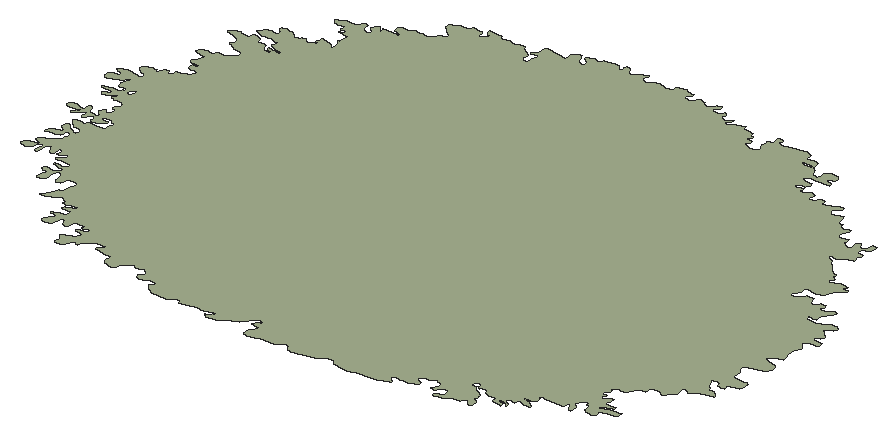
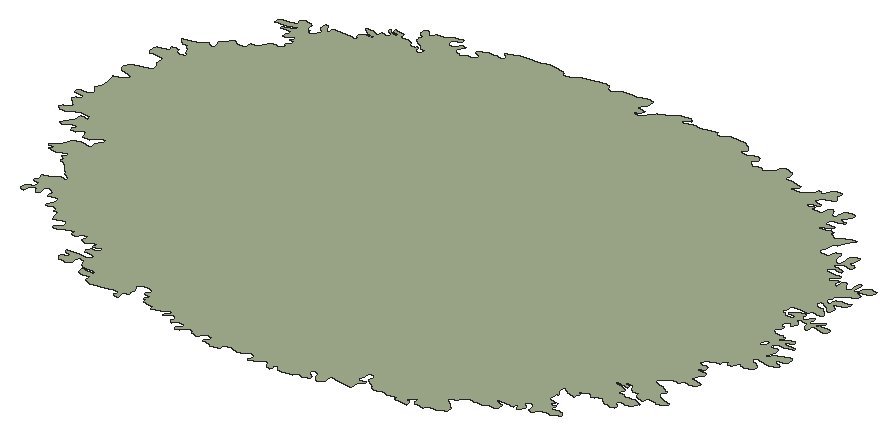
# SketchUp Ruby script. Lengths in inches.
U = 1.inch
M = Sketchup.active_model
def pt(a) = Geom::Point3d.new(a.map { |v| v * U })
def face(e, loops, mat)
  f = e.add_face(loops[0].map { |a| pt(a) })
  loops[1..].each { |l| e.add_face(l.map { |a| pt(a) }).erase! }
  f.material = f.back_material = mat if mat
  f
end
# faces: each face lists its corners as indices into pts; further lists are holes
def faces(e, pts, list, mat = nil) = list.each { |f| face(e, (f[0].is_a?(Array) ? f : [f]).map { |l| l.map { |i| pts[i] } }, mat) }
# xy, xz, yz: faces in a plane at the given z, y or x. An outline is a flat list of corners, or four numbers for a rectangle; further outlines are holes
def ring(l) = l.size == 4 ? [[l[0], l[1]], [l[2], l[1]], [l[2], l[3]], [l[0], l[3]]] : l.each_slice(2).to_a
def flat(e, list, mat, &to3) = list.each { |f| face(e, (f[0].is_a?(Array) ? f : [f]).map { |l| ring(l).map { |u, v| to3.(u, v) } }, mat) }
def xy(e, z, list, mat = nil) = flat(e, list, mat) { |x, y| [x, y, z] }
def xz(e, y, list, mat = nil) = flat(e, list, mat) { |x, z| [x, y, z] }
def yz(e, x, list, mat = nil) = flat(e, list, mat) { |y, z| [x, y, z] }
def lines(e, pts, list) = list.each { |a, b| e.add_line(pt(pts[a]), pt(pts[b])) }
# prism: a flat outline (further loops are holes) pulled along v
def prism(e, loops, v, mat = nil)
  f = face(e, loops, mat); d = Geom::Vector3d.new(v.map { |x| x * U })
  f.pushpull(f.normal.samedirection?(d) ? d.length : -d.length)
end
def box(e, o, s, mat = nil) = prism(e, [[o, [o[0] + s[0], o[1], o[2]], [o[0] + s[0], o[1] + s[1], o[2]], [o[0], o[1] + s[1], o[2]]]], [0, 0, s[2]], mat)
def at(x, y, z, deg = 0) = Geom::Transformation.translation(pt([x, y, z])) * Geom::Transformation.rotation(ORIGIN, Z_AXIS, deg.degrees)
def axes(o, x, y, z) = Geom::Transformation.new([*x, 0, *y, 0, *z, 0, *pt(o).to_a, 1])
def part(name) = M.definitions.add(name)
# library, detail: a bought-in or finely detailed component or shape, given as its bounding box
def library(name, o, s) = part(name).tap { |d| box(d.entities, o, s) }
def detail(e, o, s) = box(e.add_group.entities, o, s)
def put(e, d, t, mat = nil) = e.add_instance(d, t).tap { |i| i.material = mat if mat }
def group(e, t, mat = nil) = e.add_group.tap { |g| g.transformation = t; g.material = mat if mat }.entities
root = M.entities
M.materials.add("Boxwoodplan").color = [166, 177, 144]
xy(root,9.058,[[[69.667,67.129,69.556,67.133,69.461,67.159,69.405,67.215,69.403,67.317,69.429,67.382,69.493,67.445,69.542,67.509,69.6,67.606,69.414,67.635,69.324,67.644,69.344,67.732,69.43,67.79,69.461,67.8,69.456,67.846,69.367,67.877,69.251,67.837,69.154,67.706,69.011,67.551,68.85,67.464,68.745,67.441,68.684,67.416,68.668,67.373,68.524,67.281,68.33,67.251,68.241,67.26,68.161,67.306,68.161,67.328,68.206,67.359,68.297,67.437,68.365,67.483,68.276,67.498,68.163,67.48,68.043,67.436,67.947,67.445,67.85,67.454,67.753,67.447,67.626,67.403,67.426,67.356,67.337,67.349,67.299,67.443,67.291,67.465,67.224,67.473,67.135,67.454,66.966,67.336,66.766,67.328,66.536,67.353,66.369,67.446,66.228,67.61,66.411,67.702,66.311,67.756,66.175,67.772,66.049,67.749,65.977,67.697,65.896,67.672,65.78,67.738,65.738,67.806,65.826,67.847,65.852,67.907,65.857,67.957,65.816,68.009,65.744,68.085,65.658,68.117,65.571,68.064,65.505,68.038,65.449,68.08,65.432,68.103,65.408,68.121,65.379,68.111,65.299,68.058,65.228,68.01,65.152,67.923,65.14,67.79,65.069,67.749,65.019,67.723,64.959,67.725,64.86,67.746,64.773,67.793,64.729,67.861,64.721,67.951,64.73,68.018,64.743,68.04,64.724,68.08,64.51,68.1,64.578,68.135,64.552,68.136,64.459,68.13,64.289,68.146,64.212,68.173,64.195,68.206,64.21,68.224,64.335,68.314,64.333,68.371,64.248,68.393,64.089,68.39,63.958,68.319,63.861,68.233,63.786,68.199,63.739,68.172,63.738,68.154,63.774,68.101,63.758,68.046,63.688,68.081,63.624,68.121,63.563,68.072,63.541,68.017,63.509,67.904,63.462,67.855,63.389,67.822,63.298,67.816,63.228,67.841,63.209,67.874,63.216,67.892,63.237,67.932,63.259,67.991,63.228,68.048,63.127,68.149,63.241,68.229,63.302,68.269,63.382,68.285,63.449,68.315,63.504,68.37,63.589,68.476,63.517,68.503,63.4375,68.511,63.305,68.53,63.267,68.565,63.274,68.584,63.349,68.62,63.511,68.657,63.553,68.709,63.548,68.748,63.522,68.764,63.372,68.711,63.326,68.732,63.327,68.752,63.35,68.814,63.189,68.825,63.108,68.833,63.054,68.826,63.047,68.806,63.031,68.71,63.016,68.642,62.974,68.591,62.927,68.578,62.908,68.594,62.849,68.639,62.804,68.757,62.765,68.783,62.738,68.784,62.684,68.777,62.677,68.757,62.675,68.641,62.621,68.523,62.56,68.449,62.48,68.419,62.401,68.422,62.355,68.448,62.322,68.506,62.322,68.564,62.376,68.677,62.49,68.784,62.51,68.803,62.497,68.823,62.47,68.829,62.39,68.847,62.309,68.86,62.282,68.875,62.289,68.895,62.309,68.914,62.458,68.982,62.62,69.005,62.662,69.108,62.635,69.169,62.588,69.191,62.561,69.187,62.398,69.168,62.357,69.2,62.364,69.22,62.391,69.279,62.549,69.334,62.721,69.403,62.769,69.442,62.756,69.463,62.659,69.436,62.488,69.417,62.344,69.372,62.255,69.386,62.228,69.392,62.234,69.412,62.255,69.426,62.31,69.47,62.282,69.507,62.255,69.503,62.172,69.511,62.117,69.56,62.103,69.601,62.076,69.597,61.993,69.575,61.836,69.489,61.687,69.413,61.613,69.38,61.558,69.392,61.571,69.412,61.59,69.452,61.617,69.469,61.641,69.55,61.691,69.65,61.723,69.759,61.774,69.812,61.847,69.852,61.891,69.972,61.913,70.112,61.933,70.227,61.929,70.285,61.884,70.321,61.803,70.335,61.717,70.335,61.643,70.31,61.633,70.245,61.634,70.184,61.601,70.124,61.513,70.087,61.456,70.096,61.418,70.155,61.407,70.216,61.381,70.337,61.376,70.4,61.335,70.453,61.308,70.475,61.27,70.491,61.211,70.479,61.177,70.46,61.175,70.428,61.167,70.366,61.17,70.229,61.195,70.167,61.187,70.103,61.136,70.038,61.088,70.01,61.05,69.998,61.012,70.003,60.97,70.011,60.952,70.039,60.948,70.166,60.969,70.223,61.014,70.276,61.03,70.306,61.022,70.334,60.965,70.34,60.883,70.346,60.846,70.362,60.823,70.39,60.82,70.453,60.835,70.483,60.87,70.499,61.042,70.472,61.121,70.497,61.17,70.526,61.231,70.573,61.244,70.636,61.221,70.662,61.177,70.664,61.1,70.67,61.008,70.681,60.907,70.717,60.888,70.746,60.894,70.76,60.913,70.763,60.973,70.775,61.148,70.761,61.238,70.787,61.25,70.844,61.224,70.907,61.152,70.946,61.073,70.953,60.96,70.946,60.86,70.921,60.777,70.939,60.773,70.968,60.793,70.997,60.84,71.054,60.906,71.11,60.959,71.19,60.951,71.224,60.906,71.241,60.841,71.24,60.723,71.14,60.683,71.141,60.649,71.161,60.671,71.22,60.687,71.287,60.644,71.35,60.604,71.366,60.584,71.367,60.578,71.352,60.582,71.306,60.579,71.164,60.538,71.102,60.499,71.108,60.464,71.131,60.366,71.262,60.342,71.327,60.317,71.355,60.302,71.344,60.246,71.293,60.211,71.234,60.231,71.103,60.236,71.037,60.216,70.971,60.166,70.962,60.132,70.978,60.122,71.023,60.142,71.155,60.151,71.233,60.151,71.27,60.136,71.282,60.121,71.272,60.042,71.237,60.002,71.183,59.993,71.12,59.954,71.077,59.817,70.987,59.777,70.977,59.733,70.986,59.653,71.026,59.633,71.056,59.637,71.089,59.67,71.151,59.767,71.237,59.857,71.263,59.947,71.263,60.042,71.267,59.981,71.318,59.83,71.404,59.813,71.466,59.866,71.503,59.958,71.573,60.077,71.635,60.195,71.709,60.231,71.723,60.257,71.746,60.283,71.789,60.286,71.882,60.319,72.003,60.32,72.065,60.299,72.086,60.277,72.095,60.214,72.109,60.181,72.104,60.177,72.088,60.189,71.996,60.147,71.934,60.099,71.899,60.022,71.871,59.951,71.858,59.79,71.833,59.755,71.839,59.742,71.853,59.742,71.86,59.751,71.901,59.768,71.947,59.81,71.995,59.879,72.042,59.938,72.063,59.996,72.065,60.035,72.068,60.055,72.075,60.078,72.096,60.073,72.121,60.019,72.151,59.951,72.207,59.919,72.264,59.915,72.331,59.928,72.382,59.98,72.426,60.006,72.432,60.017,72.425,60.037,72.411,60.08,72.35,60.129,72.304,60.257,72.226,60.331,72.192,60.366,72.177,60.386,72.184,60.41,72.206,60.417,72.222,60.428,72.263,60.413,72.32,60.37,72.366,60.338,72.389,60.304,72.401,60.244,72.401,60.17,72.404,60.127,72.446,60.041,72.519,59.982,72.569,59.943,72.617,59.944,72.646,59.968,72.671,60.024,72.698,60.059,72.703,60.1,72.7,60.16,72.679,60.222,72.677,60.258,72.684,60.292,72.726,60.341,72.757,60.4,72.764,60.471,72.764,60.625,72.771,60.765,72.792,60.798,72.808,60.799,72.826,60.793,72.868,60.781,72.913,60.792,72.957,60.822,73.06,60.809,73.083,60.786,73.097,60.729,73.126,60.676,73.164,60.603,73.192,60.53,73.195,60.48,73.184,60.459,73.17,60.434,73.119,60.439,73.098,60.45,73.093,60.474,73.088,60.625,73.076,60.651,73.071,60.656,73.0625,60.647,73.046,60.607,73.007,60.562,72.964,60.497,72.928,60.435,72.884,60.363,72.849,60.326,72.852,60.306,72.863,60.281,72.9,60.274,72.995,60.257,73.02,60.275,73.034,60.281,73.077,60.275,73.088,60.264,73.088,60.249,73.087,60.223,73.083,60.191,73.076,60.173,73.065,60.092,72.97,60.06,72.915,60.029,72.892,60.006,72.895,59.98,72.916,59.971,72.932,59.965,72.973,59.994,73.057,59.999,73.102,59.99,73.13,59.97,73.137,59.932,73.128,59.912,73.114,59.866,73.064,59.744,72.957,59.708,72.932,59.682,72.927,59.645,72.935,59.633,72.951,59.724,73.057,59.787,73.102,59.801,73.129,59.8,73.145,59.791,73.152,59.78,73.148,59.765,73.143,59.734,73.131,59.65,73.108,59.483,73.089,59.41,73.096,59.362,73.121,59.34,73.149,59.339,73.165,59.356,73.217,59.404,73.264,59.464,73.281,59.535,73.284,59.609,73.266,59.737,73.223,59.823,73.197,59.834,73.201,59.834,73.22,59.825,73.239,59.8,73.287,59.799,73.342,59.806,73.407,59.818,73.437,59.835,73.45,59.884,73.413,59.923,73.363,59.95,73.317,59.96,73.255,59.972,73.204,59.987,73.176,60.01,73.175,60.145,73.157,60.218,73.144,60.253,73.14,60.271,73.154,60.286,73.202,60.231,73.244,60.172,73.309,60.155,73.335,60.155,73.352,60.189,73.46,60.219,73.483,60.246,73.489,60.261,73.477,60.27,73.459,60.299,73.414,60.31,73.39,60.322,73.391,60.343,73.404,60.423,73.482,60.44,73.528,60.441,73.579,60.427,73.611,60.406,73.623,60.343,73.646,60.303,73.666,60.295,73.687,60.311,73.736,60.367,73.773,60.401,73.795,60.414,73.816,60.422,73.869,60.42,73.916,60.325,73.992,60.181,74.014,60.119,74.031,60.084,74.013,60.056,74.014,59.987,74.031,59.968,74.058,59.977,74.082,60.103,74.185,60.097,74.217,60.075,74.233,60.03,74.225,60.001,74.216,59.875,74.154,59.835,74.107,59.786,74.063,59.717,74.049,59.689,74.05,59.642,74.102,59.67,74.126,59.6875,74.165,59.719,74.188,59.813,74.22,59.858,74.25,59.847,74.281,59.834,74.283,59.824,74.276,59.798,74.27,59.759,74.273,59.624,74.284,59.477,74.3125,59.453,74.327,59.459,74.347,59.484,74.375,59.697,74.435,59.76,74.434,59.821,74.419,59.881,74.391,59.908,74.393,59.914,74.403,59.963,74.48,59.987,74.495,59.993,74.515,59.993,74.583,59.982,74.593,59.969,74.591,59.911,74.591,59.854,74.585,59.807,74.568,59.783,74.576,59.762,74.596,59.737,74.63,59.717,74.718,59.728,74.806,59.758,74.848,59.764,74.88,59.777,74.923,59.814,74.944,59.81,74.99,59.788,75.026,59.699,75.003,59.681,74.969,59.682,74.95,59.685,74.886,59.605,74.839,59.464,74.745,59.308,74.7,59.224,74.725,59.182,74.778,59.173,74.904,59.301,74.99,59.384,75.003,59.427,75.027,59.451,75.061,59.45,75.081,59.364,75.112,59.291,75.138,59.229,75.194,59.264,75.249,59.34,75.278,59.436,75.312,59.501,75.311,59.68,75.267,59.772,75.246,59.857,75.25,59.908,75.269,59.914,75.289,59.898,75.355,59.837,75.407,59.792,75.415,59.68,75.485,59.633,75.527,59.619,75.564,59.612,75.617,59.612,75.644,59.625,75.659,59.667,75.695,59.718,75.709,59.832,75.741,59.863,75.751,59.903,75.75,59.953,75.746,59.966,75.733,59.981,75.703,59.995,75.689,60.005,75.689,60.033,75.692,60.049,75.704,60.07,75.754,60.098,75.787,60.114,75.81,60.117,75.835,60.133,75.86,60.153,75.872,60.201,75.884,60.24,75.877,60.261,75.833,60.265,75.781,60.282,75.755,60.303,75.754,60.345,75.796,60.37,75.838,60.384,75.942,60.4,75.968,60.432,75.975,60.464,75.974,60.483,75.963,60.504,75.94,60.536,75.94,60.589,75.961,60.633,76.007,60.647,76.032,60.636,76.046,60.696,76.043,60.725,76.046,60.741,76.066,60.746,76.114,60.78,76.155,60.814,76.2,60.76,76.243,60.693,76.272,60.656,76.271,60.623,76.261,60.581,76.249,60.539,76.255,60.517,76.271,60.496,76.295,60.473,76.397,60.486,76.423,60.491,76.439,60.501,76.443,60.606,76.463,60.652,76.472,60.67,76.483,60.66,76.486,60.574,76.514,60.508,76.526,60.48,76.519,60.445,76.52,60.409,76.52,60.373,76.532,60.335,76.582,60.317,76.611,60.317,76.642,60.332,76.663,60.361,76.678,60.392,76.697,60.4,76.725,60.43,76.782,60.457,76.836,60.463,76.89,60.456,76.917,60.416,76.928,60.338,76.954,60.165,77.001,60.129,77.018,60.112,77.042,60.148,77.097,60.192,77.131,60.238,77.159,60.293,77.178,60.345,77.1875,60.398,77.184,60.453,77.16,60.508,77.162,60.535,77.167,60.548,77.187,60.565,77.228,60.602,77.264,60.623,77.282,60.649,77.284,60.718,77.267,60.78,77.256,60.806,77.253,60.83,77.268,60.917,77.336,61.004,77.401,61.058,77.498,61.054,77.542,61.013,77.579,60.896,77.617,60.77,77.647,60.684,77.719,60.626,77.755,60.557,77.776,60.53,77.788,60.516,77.808,60.538,77.855,60.586,77.896,60.584,77.981,60.534,78.06,60.404,78.116,60.116,78.212,60.095,78.246,60.167,78.31,60.288,78.362,60.393,78.367,60.45,78.353,60.494,78.327,60.543,78.317,60.596,78.326,60.657,78.337,60.686,78.368,60.701,78.448,60.718,78.483,60.772,78.482,60.829,78.471,60.877,78.451,60.944,78.392,60.968,78.358,60.982,78.318,60.983,78.249,60.989,78.245,60.998,78.249,61.025,78.262,61.076,78.268,61.165,78.271,61.245,78.235,61.279,78.17,61.304,78.092,61.374,78.047,61.414,78.035,61.432,78.034,61.459,78.043,61.554,78.05,61.571,78.055,61.551,78.071,61.488,78.095,61.436,78.099,61.398,78.118,61.379,78.152,61.376,78.164,61.379,78.184,61.394,78.191,61.429,78.192,61.471,78.185,61.577,78.156,61.692,78.152,61.744,78.159,61.762,78.162,61.788,78.173,61.744,78.203,61.703,78.213,61.617,78.228,61.559,78.242,61.518,78.244,61.496,78.248,61.471,78.263,61.419,78.289,61.372,78.315,61.35,78.348,61.36,78.404,61.389,78.442,61.43,78.471,61.39,78.502,61.335,78.517,61.292,78.52,61.237,78.528,61.206,78.555,61.188,78.591,61.174,78.6,61.145,78.599,61.029,78.571,60.977,78.557,60.928,78.559,60.88,78.562,60.831,78.578,60.783,78.595,60.743,78.602,60.657,78.65,60.682,78.662,60.684,78.669,60.695,78.709,60.711,78.745,60.737,78.782,60.768,78.814,60.812,78.839,60.865,78.862,60.91,78.873,61.016,78.867,61.093,78.862,61.126,78.858,61.137,78.857,61.137,78.87,61.129,78.912,61.108,78.956,61.072,78.995,61.029,79.026,60.996,79.073,60.998,79.096,61.009,79.117,61.056,79.147,61.108,79.17,61.135,79.169,61.161,79.163,61.215,79.148,61.283,79.142,61.33,79.127,61.354,79.114,61.372,79.095,61.416,79.055,61.455,79.02,61.5,78.989,61.556,78.976,61.61,78.981,61.655,79.01,61.687,79.046,61.736,79.084,61.762,79.083,61.784,79.069,61.825,79.027,61.872,78.994,62,79.019,62.074,79.037,62.115,79.065,62.121,79.085,62.1,79.102,62.049,79.124,62.039,79.147,62.047,79.169,62.063,79.214,62.07,79.273,62.074,79.299,62.097,79.315,62.124,79.316,62.154,79.308,62.196,79.288,62.33,79.248,62.391,79.226,62.43,79.193,62.457,79.153,62.472,79.13,62.479,79.123,62.488,79.126,62.496,79.131,62.529,79.176,62.535,79.212,62.525,79.315,62.503,79.362,62.479,79.397,62.444,79.436,62.434,79.466,62.445,79.477,62.456,79.475,62.478,79.476,62.477,79.484,62.482,79.508,62.475,79.549,62.46,79.705,62.462,79.782,62.347,79.802,62.25,79.804,62.1875,79.8125,62.17,79.819,62.156,79.83,62.169,79.839,62.282,79.882,62.316,79.911,62.315,79.924,62.292,79.948,62.256,79.952,62.203,79.94,62.155,79.918,62.138,79.919,62.123,79.945,62.149,80.028,62.152,80.069,62.151,80.082,62.127,80.103,62.038,80.085,61.925,80.088,61.816,80.105,61.755,80.185,61.753,80.213,61.791,80.25,61.887,80.303,61.936,80.33,61.99,80.335,62.115,80.332,62.206,80.337,62.266,80.346,62.306,80.384,62.346,80.418,62.354,80.461,62.38,80.5,62.436,80.513,62.473,80.509,62.516,80.475,62.527,80.389,62.534,80.3,62.558,80.257,62.613,80.231,62.705,80.212,62.76,80.234,62.778,80.276,62.755,80.319,62.708,80.355,62.652,80.442,62.688,80.521,62.762,80.603,62.781,80.606,62.805,80.576,62.824,80.528,62.898,80.447,62.926,80.421,62.917,80.475,62.899,80.57,62.955,80.587,63.016,80.582,63.143,80.578,63.256,80.575,63.378,80.557,63.396,80.557,63.384,80.587,63.333,80.629,63.203,80.681,63.165,80.689,63.142,80.735,63.144,80.826,63.179,80.871,63.228,80.896,63.344,80.901,63.441,80.91,63.536,80.977,63.662,80.982,63.778,80.971,63.874,80.953,63.995,80.946,64.038,80.991,64.051,81.038,64.094,81.133,64.183,81.187,64.303,81.244,64.315,81.26,64.298,81.294,64.257,81.332,64.15,81.413,64.082,81.487,64.024,81.528,63.967,81.57,63.998,81.577,63.997,81.591,63.992,81.612,63.981,81.679,63.984,81.709,64.019,81.744,64.102,81.785,64.185,81.821,64.223,81.827,64.279,81.826,64.366,81.816,64.389,81.808,64.413,81.81,64.445,81.843,64.497,81.918,64.533,81.932,64.59,81.936,64.692,81.93,64.788,81.898,64.82,81.877,64.849,81.835,64.85,81.765,64.853,81.736,64.858,81.715,64.881,81.704,64.934,81.715,64.979,81.745,65.041,81.798,65.066,81.822,65.087,81.834,65.1,81.85,65.015,81.897,64.977,81.913,64.934,81.956,64.909,82.036,64.91,82.067,64.968,82.083,65.16,82.055,65.257,82.039,65.292,82.026,65.292,81.98,65.302,81.952,65.362,81.948,65.466,81.962,65.568,81.975,65.61,81.971,65.657,81.957,65.684,81.934,65.709,81.933,65.734,81.943,65.878,81.972,65.919,81.981,65.971,81.987,66.007,81.984,66.052,81.957,66.082,81.886,66.108,81.863,66.153,81.844,66.193,81.833,66.233,81.808,66.285,81.753,66.339,81.696,66.326,81.619,66.319,81.545,66.333,81.515,66.364,81.485,66.391,81.461,66.438,81.453,66.474,81.45,66.519,81.481,66.532,81.512,66.533,81.553,66.521,81.628,66.558,81.787,66.547,81.817,66.529,81.829,66.505,81.833,66.466,81.834,66.414,81.828,66.378,81.826,66.331,81.835,66.306,81.858,66.313,81.88,66.341,81.896,66.38,81.91,66.425,81.937,66.45,82.013,66.454,82.178,66.454,82.21,66.477,82.228,66.503,82.233,66.602,82.222,66.801,82.201,66.892,82.19,66.981,82.169,67.068,82.153,67.119,82.147,67.114,82.355,67.182,82.427,67.267,82.486,67.321,82.477,67.349,82.441,67.397,82.37,67.42,82.297,67.428,82.26,67.426,82.241,67.453,82.206,67.558,82.173,67.61,82.173,67.649,82.204,67.652,82.279,67.549,82.36,67.471,82.419,67.483,82.453,67.527,82.49,67.621,82.541,67.671,82.55,67.752,82.538,67.856,82.537,67.879,82.615,68.089,82.643,68.189,82.661,68.297,82.647,68.376,82.578,68.409,82.543,68.436,82.541,68.476,82.568,68.474,82.643,68.465,82.685,68.478,82.72,68.528,82.729,68.583,82.715,68.654,82.621,68.675,82.548,68.708,82.513,68.757,82.498,68.808,82.503,68.854,82.53,68.942,82.613,69.023,82.668,69.125,82.715,69.173,82.7,69.187,82.663,69.135,82.592,69.109,82.557,69.117,82.515,69.206,82.457,69.306,82.443,69.356,82.452,69.406,82.498,69.484,82.566,69.599,82.581,69.714,82.553,69.745,82.523,69.822,82.492,69.922,82.511,70.004,82.565,70.004,82.678,70.061,82.721,70.174,82.745,70.279,82.74,70.36,82.681,70.506,82.66,70.56,82.651,70.566,82.614,70.492,82.546,70.459,82.473,70.471,82.437,70.543,82.396,70.645,82.401,70.698,82.433,70.718,82.472,70.738,82.544,70.787,82.567,70.811,82.579,70.862,82.579,70.965,82.541,71.008,82.47,71.094,82.417,71.224,82.447,71.259,82.478,71.265,82.52,71.305,82.603,71.412,82.622,71.442,82.592,71.448,82.55,71.395,82.466,71.347,82.448,71.32,82.413,71.38,82.349,71.511,82.337,71.602,82.373,71.669,82.444,71.694,82.45,71.703,82.433,71.721,82.392,71.745,82.357,71.734,82.301,71.714,82.257,71.732,82.222,71.821,82.179,71.929,82.184,71.984,82.203,72.035,82.258,72.052,82.273,72.054,82.255,72.041,82.212,71.968,82.132,71.934,82.102,71.945,82.066,71.992,82.047,72.05,82.048,72.146,82.088,72.228,82.146,72.448,82.225,72.47,82.153,72.493,82.123,72.544,82.118,72.66,82.11,72.784,82.084,72.799,82.013,72.822,81.983,72.868,81.964,72.891,81.93,72.877,81.892,72.85,81.795,72.967,81.773,73.013,81.755,73.023,81.72,72.949,81.65,72.935,81.613,72.951,81.579,73.027,81.527,73.13,81.5,73.231,81.496,73.343,81.563,73.385,81.639,73.327,81.71,73.294,81.779,73.314,81.885,73.323,81.922,73.294,81.956,73.29,81.992,73.332,82.018,73.433,82.022,73.422,82.122,73.38,82.274,73.43,82.287,73.495,82.275,73.548,82.256,73.579,82.199,73.529,82.131,73.533,82.095,73.579,82.076,73.687,82.076,73.817,82.111,74.324,82.178,74.37,82.168,74.416,82.145,74.462,82.121,74.496,82.097,74.527,82.027,74.51,81.935,74.714,81.949,74.779,81.943,74.864,81.911,74.901,81.805,74.886,81.757,74.87,81.724,74.829,81.717,74.659,81.749,74.595,81.755,74.552,81.755,74.532,81.749,74.529,81.733,74.557,81.685,74.598,81.666,74.645,81.666,74.818,81.681,74.887,81.683,74.971,81.648,75.008,81.609,75.039,81.546,75.107,81.437,75.186,81.398,75.271,81.394,75.302,81.435,75.296,81.518,75.278,81.571,75.285,81.637,75.326,81.687,75.427,81.719,75.536,81.732,75.625,81.701,75.673,81.659,75.707,81.597,75.708,81.551,75.646,81.495,75.58,81.482,75.539,81.471,75.507,81.437,75.511,81.407,75.56,81.389,75.658,81.363,75.729,81.339,75.749,81.306,75.737,81.275,75.683,81.247,75.596,81.24,75.434,81.233,75.347,81.222,75.258,81.256,75.194,81.269,75.112,81.251,75.056,81.208,75.054,81.143,75.112,81.103,75.199,81.081,75.285,81.066,75.332,81.066,75.366,81.046,75.387,81.003,75.37,80.938,75.335,80.89,75.307,80.866,75.262,80.854,75.12,80.834,75.1,80.829,75.091,80.784,75.095,80.751,75.14,80.732,75.207,80.731,75.248,80.731,75.298,80.746,75.361,80.778,75.375,80.712,75.346,80.665,75.339,80.635,75.378,80.617,75.439,80.622,75.521,80.67,75.577,80.711,75.605,80.736,75.643,80.721,75.707,80.704,75.776,80.651,75.772,80.603,75.729,80.537,75.696,80.472,75.714,80.448,75.761,80.445,75.837,80.456,75.919,80.495,75.958,80.554,76.03,80.597,76.09,80.609,76.127,80.601,76.145,80.577,76.148,80.548,76.131,80.521,76.103,80.497,76.105,80.483,76.126,80.481,76.298,80.499,76.379,80.51,76.446,80.552,76.488,80.589,76.567,80.614,76.664,80.619,76.687,80.595,76.69,80.566,76.53,80.349,76.545,80.304,76.602,80.251,76.685,80.237,76.774,80.255,76.842,80.283,76.927,80.305,76.992,80.213,77.028,79.999,77.03,79.985,77.066,79.974,77.15,79.996,77.161,79.918,77.185,79.871,77.261,79.861,77.398,79.896,77.466,79.893,77.481,79.839,77.413,79.619,77.402,79.567,77.425,79.514,77.491,79.486,77.559,79.496,77.695,79.523,77.715,79.419,77.71,79.316,77.832,79.247,77.965,79.216,77.995,79.318,77.985,79.421,77.962,79.474,77.99,79.525,78.059,79.535,78.098,79.482,78.12,79.429,78.168,79.395,78.245,79.418,78.299,79.467,78.323,79.583,78.327,79.636,78.388,79.659,78.445,79.631,78.475,79.577,78.45,79.455,78.335,79.375,78.282,79.339,78.261,79.282,78.241,79.231,78.264,79.186,78.396,79.161,78.452,79.134,78.457,79.083,78.384,78.997,78.419,78.895,78.448,78.844,78.436,78.794,78.302,78.768,78.201,78.729,78.097,78.658,78.046,78.623,77.98,78.626,77.916,78.659,77.884,78.667,77.858,78.643,77.902,78.549,78.021,78.483,78.068,78.445,78.065,78.396,78.15,78.32,78.316,78.132,78.448,78.05,78.511,78.035,78.548,77.992,78.533,77.898,78.649,77.834,78.586,77.749,78.566,77.697,78.564,77.673,78.595,77.661,78.732,77.679,78.867,77.755,78.997,77.768,79.122,77.734,79.125,77.687,79.059,77.66,79.033,77.644,79.047,77.62,79.125,77.599,79.197,77.596,79.229,77.595,79.242,77.571,79.154,77.482,78.988,77.322,78.964,77.232,78.96,77.187,78.932,77.142,78.839,77.067,78.711,77.038,78.586,77.043,78.477,77.082,78.408,77.076,78.381,77.004,78.408,76.894,78.379,76.787,78.261,76.72,78.289,76.62,78.427,76.642,78.599,76.833,78.826,76.815,78.902,76.605,78.947,76.595,79.029,76.618,79.116,76.723,79.254,76.735,79.292,76.635,79.242,76.574,79.227,76.539,79.304,76.501,79.443,76.531,79.5625,76.598,79.609,76.614,79.699,76.592,79.677,76.477,79.566,76.384,79.501,76.289,79.509,76.113,79.495,76.078,79.402,76.056,79.27,76.087,79.295,75.981,79.426,75.941,79.572,75.936,79.721,75.965,79.958,76.087,80.094,76.099,80.186,76.008,80.153,75.905,80.013,75.849,79.966,75.825,79.9375,75.766,80.041,75.675,80.192,75.515,80.159,75.414,80.043,75.359,80.007,75.335,80.045,75.274,80.189,75.269,80.319,75.247,80.331,75.145,80.258,75.089,80.125,75.078,80,75.041,79.957,74.942,80.125,74.761,80.018,74.568,80.021,74.388,80.075,74.176,80.119,74.078,79.987,74.051,79.864,74.008,79.77,73.931,79.743,73.869,79.854,73.801,80.106,73.744,80.183,73.662,80.204,73.559,80.162,73.467,80.047,73.394,79.586,73.234,79.588,73.141,79.632,73.048,79.686,72.954,79.6875,72.863,79.682,72.803,79.679,72.773,79.705,72.719,79.826,72.676,79.951,72.672,80.077,72.682,80.119,72.68,80.177,72.633,80.188,72.453,80.161,72.395,80.052,72.347,79.925,72.33,79.884,72.331,79.838,72.281,79.88,72.191,79.867,72.163,79.782,72.144,79.741,72.145,79.671,72.17,79.639,72.26,79.569,72.292,79.446,72.297,79.404,72.291,79.388,72.233,79.464,72.156,79.551,71.992,79.579,71.969,79.605,71.918,79.623,71.888,79.704,71.877,79.784,71.86,79.869,71.792,79.932,71.71,79.929,71.681,79.845,71.656,79.596,71.616,79.401,71.488,79.328,71.469,79.233,71.544,79.193,71.553,79.129,71.52,79.132,71.435,79.188,71.27,79.146,71.264,79.113,71.219,79.064,71.18,79.01,71.066,78.971,71.019,78.937,71,78.901,71.013,78.779,71.1,78.716,71.115,78.673,71.116,78.628,71.098,78.565,71.063,78.535,70.991,78.545,70.938,78.527,70.874,78.365,70.852,78.313,70.81,78.281,70.759,78.234,70.718,78.222,70.655,78.191,70.609,78.157,70.583,78.12,70.573,78.051,70.564,77.953,70.575,77.893,70.55,77.831,70.502,77.801,70.457,77.876,70.419,77.903,70.376,77.867,70.32,77.812,70.284,77.791,70.225,77.79,70.209,77.789,70.194,77.808,70.186,77.88,70.18,77.906,70.182,77.926,70.182,77.93,70.166,77.892,70.097,77.873,70.049,77.87,70.02,77.911,70.018,78.05,70.094,78.119,70.11,78.2,70.107,78.184,70.004,78.166,69.89,78.166,69.843,78.189,69.82,78.229,69.818,78.293,69.845,78.374,69.846,78.433,69.832,78.473,69.827,78.479,69.798,78.439,69.76,78.36,69.73,78.294,69.722,78.211,69.696,78.172,69.658,78.155,69.602,78.159,69.587,78.199,69.586,78.281,69.611,78.439,69.673,78.593,69.703,78.719,69.705,78.771,69.685,78.746,69.611,78.725,69.569,78.664,69.518,78.511,69.492,78.372,69.491,78.311,69.482,78.28,69.427,78.306,69.308,78.291,69.264,78.21,69.243,78.074,69.255,78.016,69.261,77.972,69.314,77.963,69.426,77.963,69.468,77.951,69.496,77.942,69.511,77.922,69.512,77.864,69.525,77.859,69.581,77.861,69.595,77.857,69.61,77.838,69.614,77.758,69.617,77.701,69.591,77.656,69.536,77.619,69.499,77.594,69.44,77.605,69.391,77.661,69.354,77.736,69.254,77.732,69.155,77.723,69.115,77.716,69.088,77.685,69.066,77.665,69.067,77.644,69.098,77.615,69.157,77.55,69.258,77.509,69.298,77.495,69.312,77.484,69.299,77.477,69.271,77.474,69.227,77.455,69.173,77.449,69.16,77.419,69.144,77.336,69.137,77.195,69.139,76.909,69.14,76.851,69.162,76.764,69.173,76.745,69.163,76.739,69.133,76.789,69.074,76.814,68.976,76.808,68.936,76.776,68.896,76.752,68.889,76.692,68.88,76.589,68.88,76.491,68.884,76.443,68.853,76.498,68.829,76.599,68.814,76.707,68.78,76.782,68.726,76.863,68.654,76.845,68.629,76.784,68.614,76.683,68.621,76.646,68.63,76.595,68.65,76.547,68.684,76.497,68.708,76.462,68.63,76.452,68.558,76.412,68.545,76.356,68.558,76.311,68.589,76.298,68.6,76.28,68.608,76.268,68.59,76.234,68.513,76.236,68.485,76.269,68.448,76.361,68.416,76.4,68.383,76.413,68.34,76.411,68.326,76.392,68.323,76.349,68.36,76.269,68.409,76.176,68.427,76.119,68.429,76.107,68.415,76.128,68.39,76.242,68.347,76.279,68.335,76.302,68.292,76.298,68.264,76.297,68.251,76.254,68.249,76.141,68.26,76.036,68.295,76.001,68.325,75.992,68.371,75.991,68.441,75.94,68.461,75.881,68.442,75.781,68.449,75.682,68.467,75.655,68.489,75.63,68.526,75.634,68.568,75.64,68.583,75.602,68.591,75.508,68.616,75.451,68.619,75.416,68.606,75.404,68.577,75.384,68.571,75.357,68.597,75.354,68.612,75.384,68.635,75.4,68.646,75.392,68.671,75.305,68.729,75.268,68.752,75.249,68.756,75.208,68.736,75.168,68.716,75.148,68.71,75.137,68.681,75.16,68.59,75.255,68.587,75.294,68.582,75.324,68.541,75.317,68.513,75.311,68.499,75.319,68.471,75.43,68.434,75.518,68.396,75.579,68.338,75.596,68.3125,75.595,68.299,75.56,68.283,75.54,68.273,75.571,68.251,75.626,68.225,75.638,68.2,75.587,68.168,75.575,68.141,75.6,68.106,75.685,68.062,75.763,67.994,75.762,67.851,75.741,67.825,75.689,67.814,75.635,67.829,75.597,67.874,75.557,67.939,75.539,67.949,75.501,67.944,75.449,67.926,75.427,67.897,75.428,67.854,75.427,67.84,75.394,67.828,75.217,67.819,75.209,67.826,75.161,67.808,75.117,67.777,75.033,67.692,74.981,67.661,74.907,67.651,74.769,67.643,74.715,67.658,74.713,67.698,74.822,67.762,74.922,67.834,74.919,67.937,74.913,67.98,74.913,67.994,74.882,68.015,74.822,68.034,74.748,68.034,74.664,67.95,74.644,67.911,74.587,67.866,74.572,67.857,74.536,67.865,74.499,67.88,74.487,67.907,74.527,67.999,74.587,68.094,74.588,68.135,74.52,68.189,74.409,68.224,74.357,68.246,74.32,68.238,74.295,68.215,74.261,68.171,74.228,68.156,74.186,68.157,74.13,68.166,74.093,68.168,74.055,68.145,73.974,68.05,73.988,68.01,74.062,67.97,74.117,67.938,74.144,67.917,74.153,67.89,74.129,67.851,74.069,67.807,73.967,67.756,73.912,67.735,73.839,67.738,73.784,67.76,73.71,67.769,73.665,67.745,73.628,67.743,73.596,67.76,73.541,67.766,73.468,67.752,73.446,67.717,73.456,67.659,73.553,67.575,73.58,67.536,73.581,67.51,73.581,67.497,73.563,67.492,73.273,67.391,72.998,67.369,72.765,67.373,72.674,67.371,72.552,67.31,72.449,67.275,72.352,67.279,72.314,67.281,72.265,67.299,72.217,67.328,72.156,67.325,72.067,67.334,71.983,67.376,71.923,67.433,71.892,67.478,71.833,67.491,71.734,67.479,71.638,67.438,71.558,67.398,71.459,67.325,71.362,67.269,71.269,67.24,71.028,67.222,70.838,67.186,70.741,67.19,70.676,67.284,70.645,67.351,70.557,67.365,70.466,67.352,70.37,67.28,70.305,67.217,70.215,67.21,70.038,67.233,69.853,67.24,69.775,67.189],[60.175,74.415,60.217,74.419,60.237,74.422,60.263,74.431,60.275,74.474,60.276,74.513,60.283,74.597,60.275,74.631,60.263,74.643,60.263,74.658,60.22,74.635,60.164,74.612,60.144,74.606,60.128,74.59,60.107,74.557,60.097,74.52,60.099,74.476,60.118,74.437,60.137,74.421]]],"Boxwoodplan")
